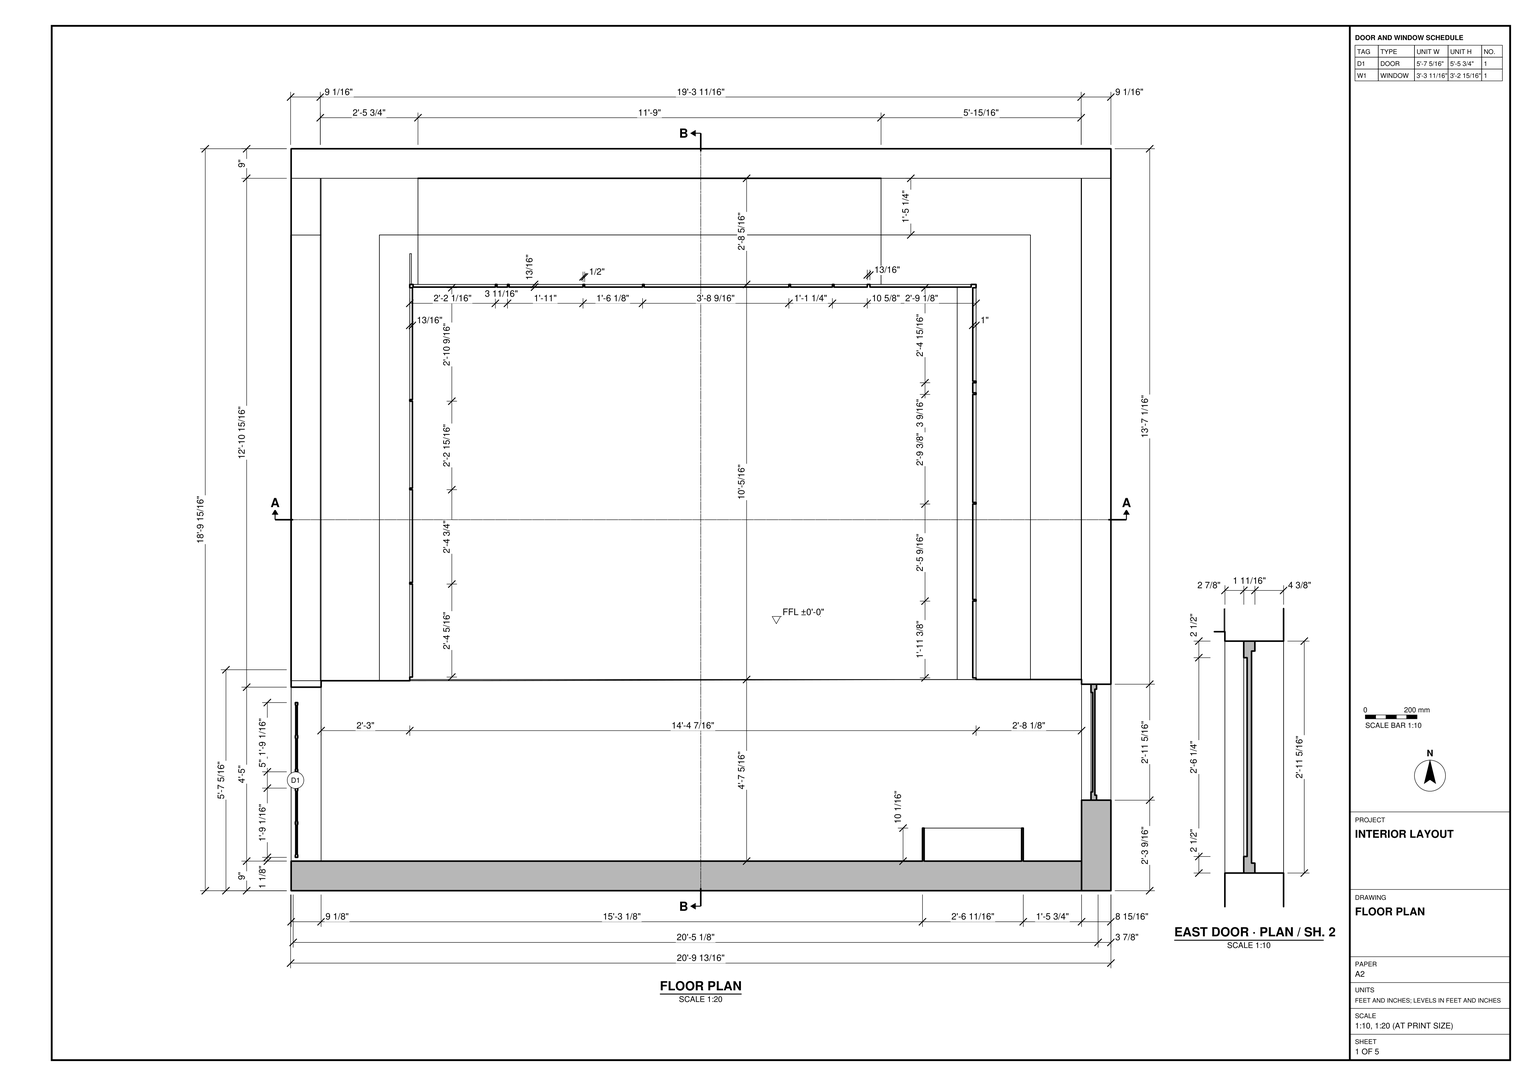
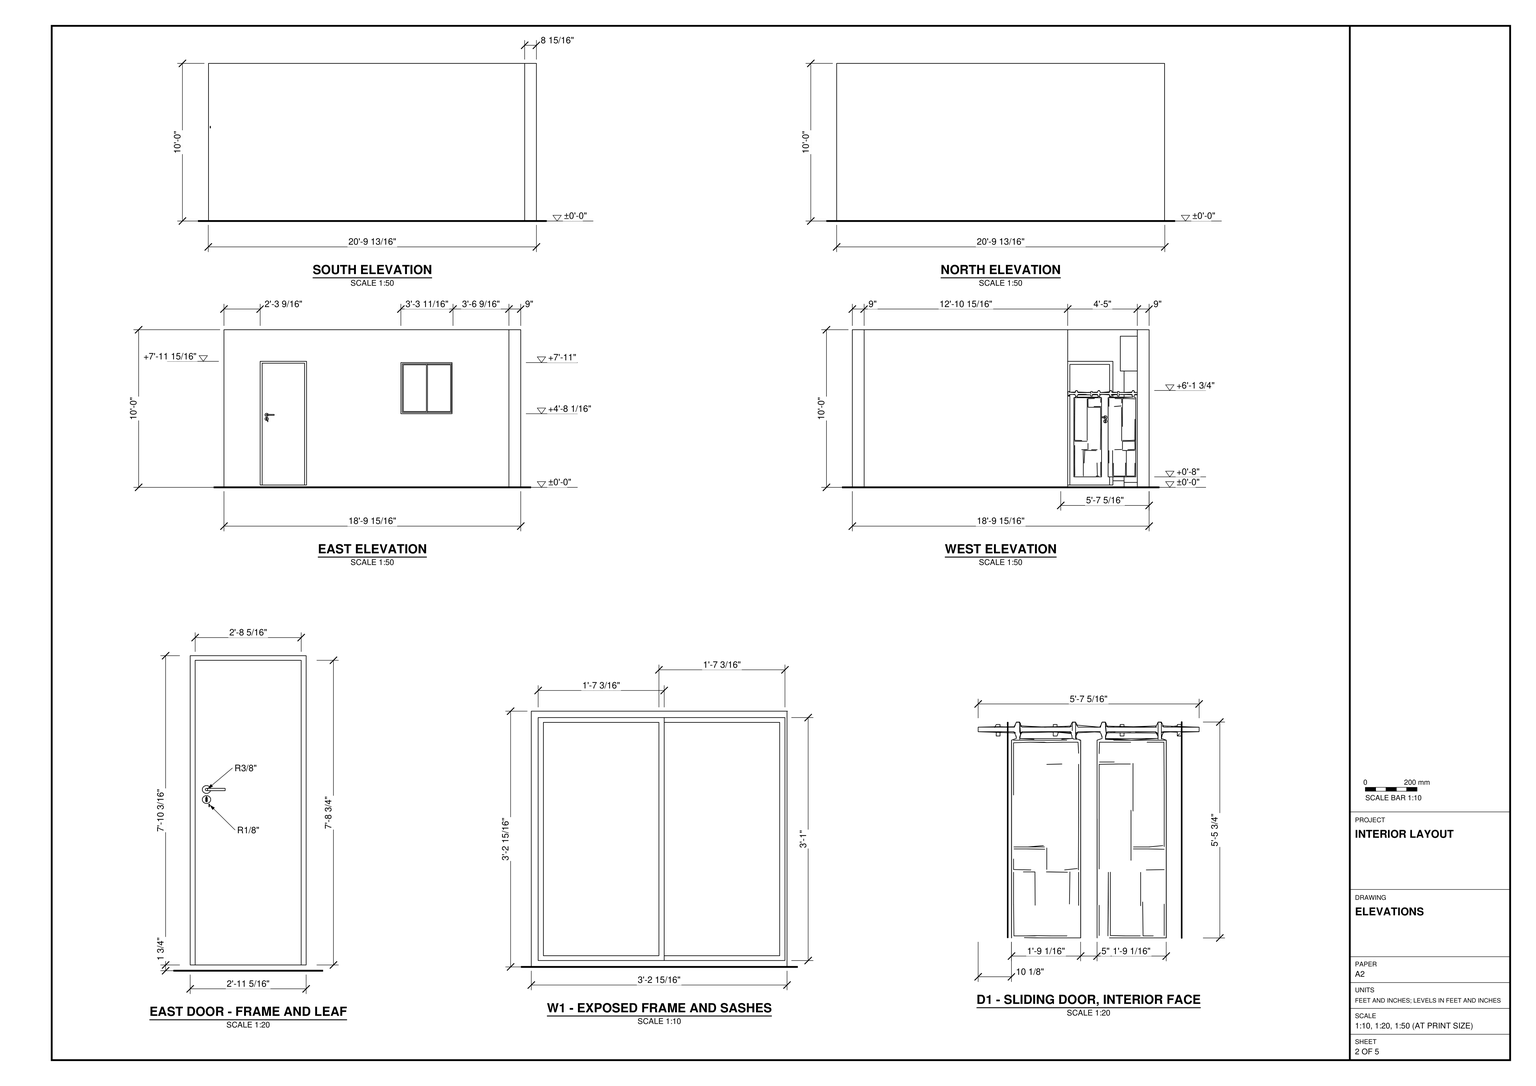
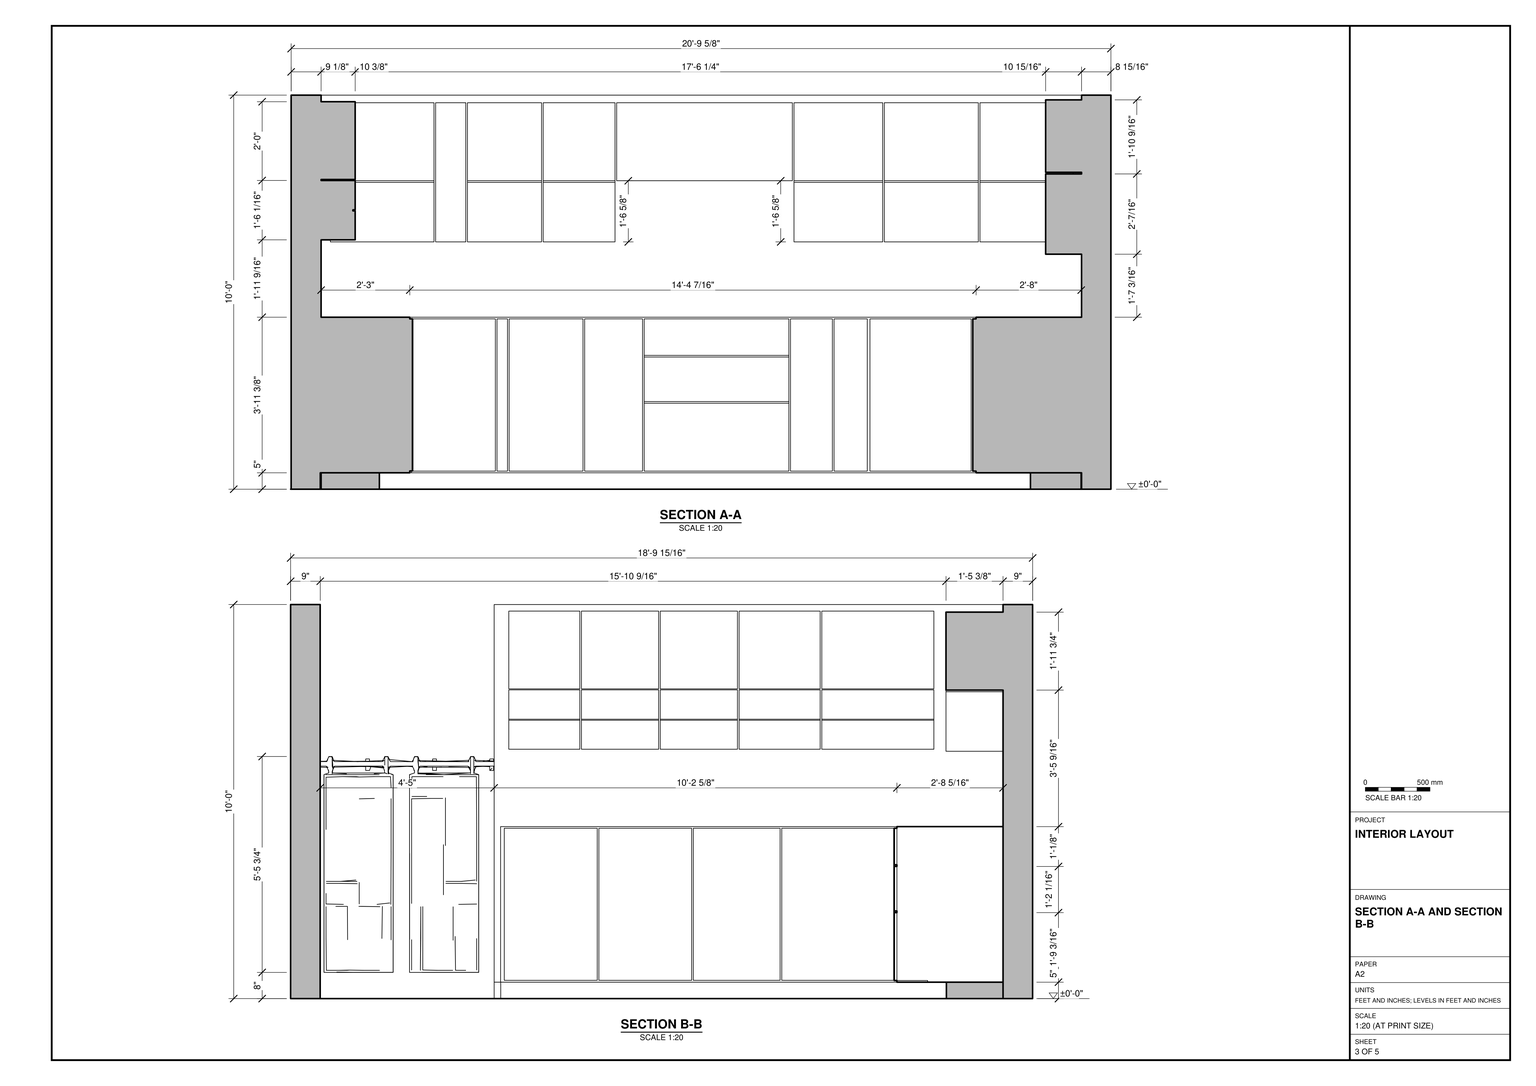
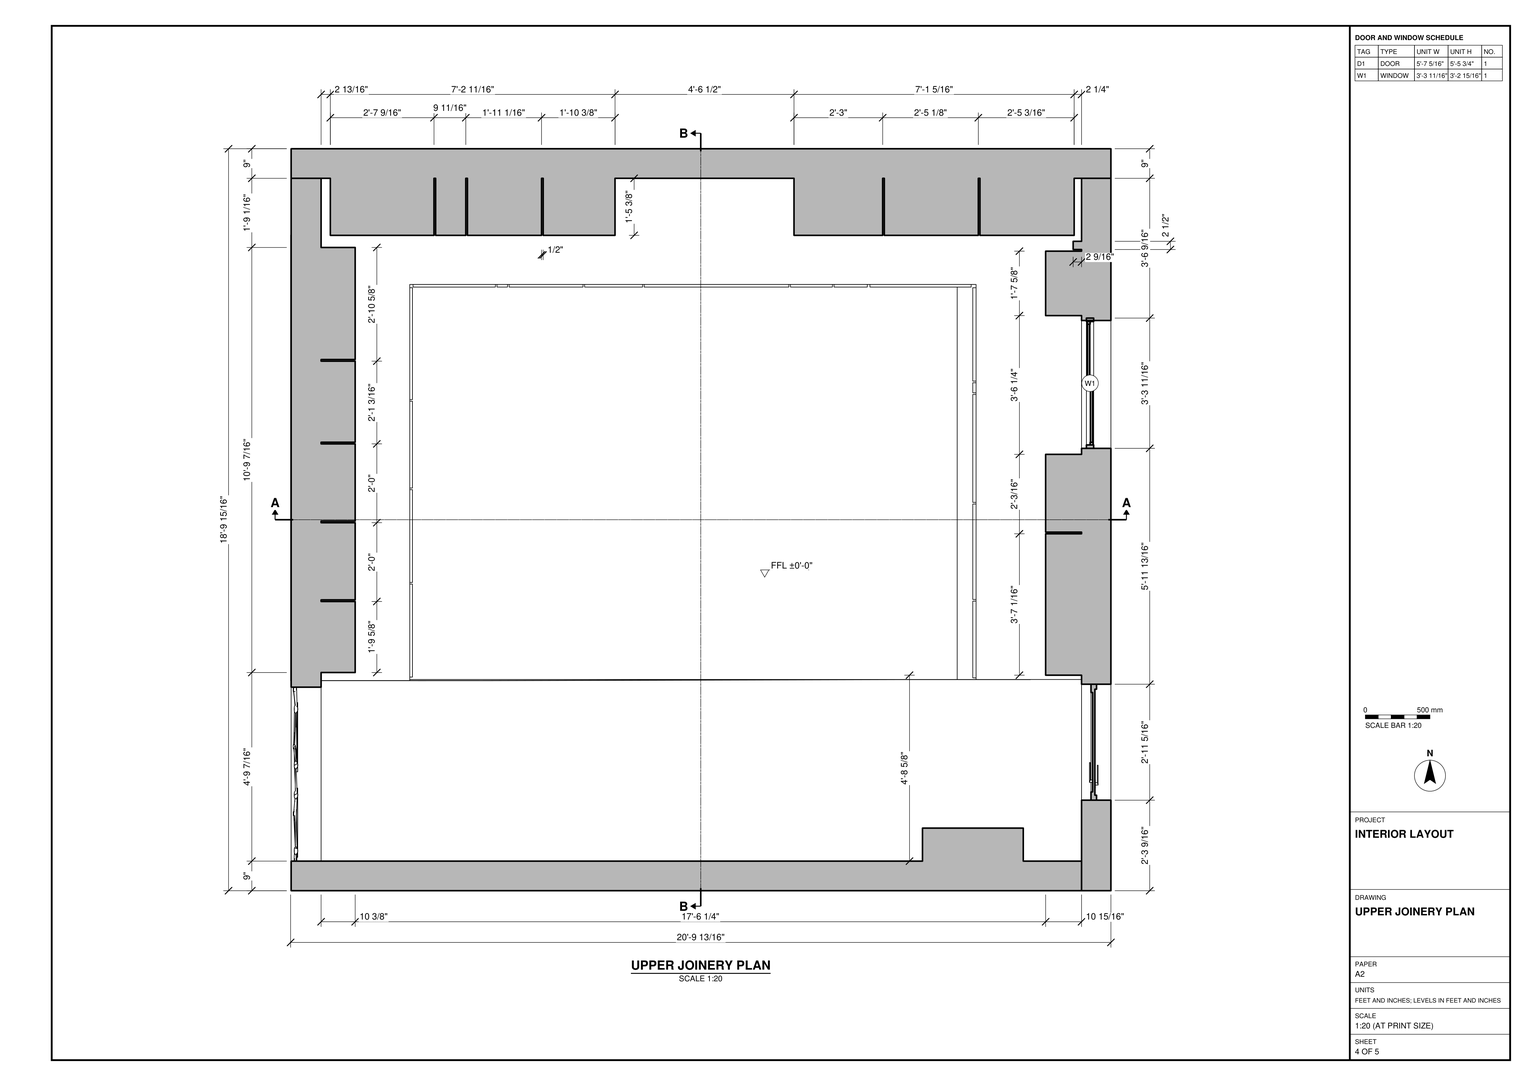
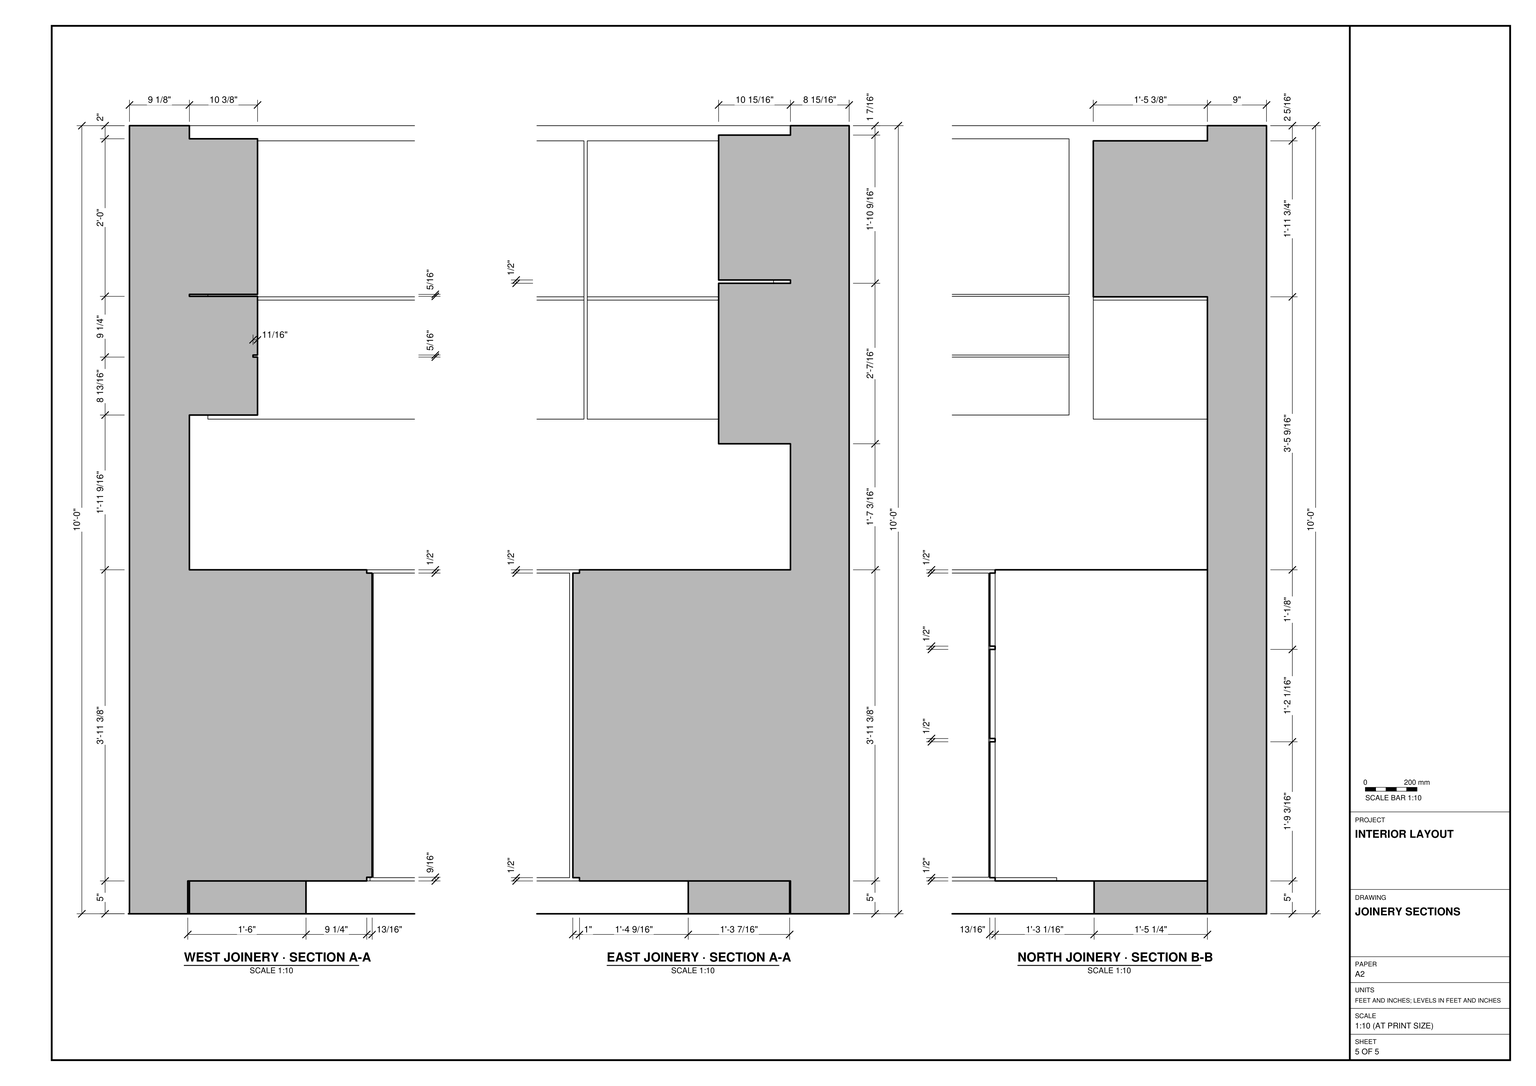
Use task_files/diagram_01.pdf to model the room and its built-in joinery in SketchUp. Work in feet and inches. Set the finished floor at ±0'-0" and make the overall shell 20'-9 13/16" east to west, 18'-9 15/16" north to south and 10'-0" high.

Lay out the perimeter walls at their drawn thicknesses. On the east wall, fit the framed single-leaf door near the south end and the two-sash window farther north. Use the elevation details for the window sill, door frame and hardware. At the south end of the west wall, model the paired sliding panels and their exposed overhead track.

Build the lower cabinetry along the north wall and return it along the west and east walls, leaving the centre open. Use the plan to set out the depths and unequal bay widths. Follow the sections for the raised plinth, lower cabinet fronts, central shelves and wall-mounted storage. Preserve the clear space between the lower and upper units rather than filling it with full-height cabinets.

Keep shell elements and each distinct furniture or joinery piece in separate groups or components. Use components for repeated parts. Any decor or loose items shown may be represented by suitable library components. Save one SketchUp model as output_files/single_room_interior_with_u_shaped_built_in_cabinetry.skp.

# SketchUp Ruby script. Lengths in inches.
U = 1.inch
M = Sketchup.active_model
def pt(a) = Geom::Point3d.new(a.map { |v| v * U })
def face(e, loops, mat)
  f = e.add_face(loops[0].map { |a| pt(a) })
  loops[1..].each { |l| e.add_face(l.map { |a| pt(a) }).erase! }
  f.material = f.back_material = mat if mat
  f
end
# faces: each face lists its corners as indices into pts; further lists are holes
def faces(e, pts, list, mat = nil) = list.each { |f| face(e, (f[0].is_a?(Array) ? f : [f]).map { |l| l.map { |i| pts[i] } }, mat) }
# xy, xz, yz: faces in a plane at the given z, y or x. An outline is a flat list of corners, or four numbers for a rectangle; further outlines are holes
def ring(l) = l.size == 4 ? [[l[0], l[1]], [l[2], l[1]], [l[2], l[3]], [l[0], l[3]]] : l.each_slice(2).to_a
def flat(e, list, mat, &to3) = list.each { |f| face(e, (f[0].is_a?(Array) ? f : [f]).map { |l| ring(l).map { |u, v| to3.(u, v) } }, mat) }
def xy(e, z, list, mat = nil) = flat(e, list, mat) { |x, y| [x, y, z] }
def xz(e, y, list, mat = nil) = flat(e, list, mat) { |x, z| [x, y, z] }
def yz(e, x, list, mat = nil) = flat(e, list, mat) { |y, z| [x, y, z] }
def lines(e, pts, list) = list.each { |a, b| e.add_line(pt(pts[a]), pt(pts[b])) }
# prism: a flat outline (further loops are holes) pulled along v
def prism(e, loops, v, mat = nil)
  f = face(e, loops, mat); d = Geom::Vector3d.new(v.map { |x| x * U })
  f.pushpull(f.normal.samedirection?(d) ? d.length : -d.length)
end
def box(e, o, s, mat = nil) = prism(e, [[o, [o[0] + s[0], o[1], o[2]], [o[0] + s[0], o[1] + s[1], o[2]], [o[0], o[1] + s[1], o[2]]]], [0, 0, s[2]], mat)
def at(x, y, z, deg = 0) = Geom::Transformation.translation(pt([x, y, z])) * Geom::Transformation.rotation(ORIGIN, Z_AXIS, deg.degrees)
def axes(o, x, y, z) = Geom::Transformation.new([*x, 0, *y, 0, *z, 0, *pt(o).to_a, 1])
def part(name) = M.definitions.add(name)
# library, detail: a bought-in or finely detailed component or shape, given as its bounding box
def library(name, o, s) = part(name).tap { |d| box(d.entities, o, s) }
def detail(e, o, s) = box(e.add_group.entities, o, s)
def put(e, d, t, mat = nil) = e.add_instance(d, t).tap { |i| i.material = mat if mat }
def group(e, t, mat = nil) = e.add_group.tap { |g| g.transformation = t; g.material = mat if mat }.entities
root = M.entities
M.materials.add("Wood_Door").color = [227, 177, 138]
M.materials.add("[Color M05]").color = [114, 114, 114]
M.materials.add("[Metal Aluminum Anodized]").color = [202, 209, 219]
M.materials.add("[Metal Corrugated Shiny]").color = [193, 193, 193]
M.materials.add("[Metal Seamed]").color = [118, 119, 115]
M.materials.add("[Translucent Glass Tinted]").color = [1, 25, 30]
M.materials["[Translucent Glass Tinted]"].alpha = 0.31
c1 = part("Group\#98")
g1 = group(c1.entities,at(-0.375,0,0),"[Metal Seamed]")
prism(g1,[[[0.375,0,0],[0.375,0,57],[0.375,26.94,57],[0.375,26.94,0]],[[0.375,25.82,55.875],[0.375,1.125,55.875],[0.375,1.125,1.125],[0.375,25.82,1.125]]],[1.5,0,0])
g2 = group(c1.entities,at(0.18,24.32,1.125),"[Translucent Glass Tinted]")
box(g2,[0,-23.19,0],[1.125,24.69,54.75])
c2 = part("Aluminium+Channel+Glass+Window")
g3 = group(c2.entities,at(-81.68,-4.64,338.57))
g4 = group(g3,at(-22.76,-500.89,-282.52),"[Metal Aluminum Anodized]")
prism(g4,[[[0,0,38.9375],[0,39.67,38.9375],[0,39.67,0],[0,0,0]],[[0,1.05,0.97],[0,38.625,0.97],[0,38.625,37.96],[0,1.05,37.96]]],[2.21,0,0])
put(g3,c1,axes([-22.54,-481.46,-281.55],[0.6,0,0],[0,0.71223,0],[0,0,0.64896]))
put(g3,c1,axes([-21.64,-499.85,-281.55],[0.6,0,0],[0,0.71223,0],[0,0,0.64896]))
c3 = library("Sliding Door 243 092",[-48.06,-2.0625,0.36],[96.12,2.0625,93.93])
c4 = part("Door lever handle")
xz(c4.entities,1.97,[[0.3,0,0.15,0.04,0.04,0.15,0,0.3,0.04,0.44,0.15,0.55,0.3,0.59,0.44,0.55,0.55,0.44,0.59,0.3,0.55,0.15,0.44,0.04]])
yz(c4.entities,4.72,[[0.3,0,0.44,0.04,0.55,0.15,0.59,0.3,0.55,0.44,0.44,0.55,0.3,0.59,0.15,0.55,0.04,0.44,0,0.3,0.04,0.15,0.15,0.04]],"[Metal Corrugated Shiny]")
p = [[0.04,1.97,0.15],[0.15,1.97,0.04],[0.15,0.15,0.04],[0.04,0.04,0.15],[4.72,0.15,0.04],[4.72,0.04,0.15],
  [0.3,1.97,0],[0.3,0.3,0],[4.72,0.3,0],[0.44,1.97,0.04],[0.44,0.44,0.04],[4.72,0.44,0.04],
  [0.55,1.97,0.15],[0.55,0.55,0.15],[4.72,0.55,0.15],[0,1.97,0.3],[0,0,0.3],[4.72,0,0.3],
  [0.59,1.97,0.3],[0.59,0.59,0.3],[4.72,0.59,0.3],[0.04,1.97,0.44],[0.04,0.04,0.44],[4.72,0.04,0.44],
  [0.55,1.97,0.44],[0.55,0.55,0.44],[4.72,0.55,0.44],[0.15,1.97,0.55],[0.15,0.15,0.55],[4.72,0.15,0.55],
  [0.44,1.97,0.55],[0.44,0.44,0.55],[4.72,0.44,0.55],[0.3,1.97,0.59],[0.3,0.3,0.59],[4.72,0.3,0.59]]
faces(c4.entities,p,[[0,1,2,3],[3,2,4,5],[1,6,7,2],[2,7,8,4],[6,9,10,7],[7,10,11,8],[9,12,13,10],[10,13,14,11],
  [15,0,3,16],[16,3,5,17],[12,18,19,13],[13,19,20,14],[21,15,16,22],[22,16,17,23],[18,24,25,19],[19,25,26,20],
  [27,21,22,28],[28,22,23,29],[24,30,31,25],[25,31,32,26],[33,27,28,34],[34,28,29,35],[30,33,34,31],[31,34,35,32]],"[Metal Corrugated Shiny]")
c5 = part("Door handle rose")
xy(c5.entities,0,[[0.72,0,1.25,0.31]],"[Metal Corrugated Shiny]")
xy(c5.entities,1.97,[[0.72,0,1.25,0.31]],"[Metal Corrugated Shiny]")
xz(c5.entities,0,[[0.72,0,1.25,0,1.71,0.26,1.97,0.72,1.97,1.25,1.71,1.71,1.25,1.97,0.72,1.97,0.26,1.71,0,1.25,0,0.72,0.26,0.26]],"[Metal Corrugated Shiny]")
yz(c5.entities,0,[[0,0.72,0.31,1.25]],"[Metal Corrugated Shiny]")
yz(c5.entities,1.97,[[0,0.72,0.31,1.25]],"[Metal Corrugated Shiny]")
p = [[0.26,0.31,0.26],[0.72,0.31,0],[0.72,0,0],[0.26,0,0.26],[1.25,0.31,0],[1.71,0.31,0.26],
  [1.71,0,0.26],[1.25,0,0],[0,0.31,0.72],[0,0,0.72],[1.97,0.31,0.72],[1.97,0,0.72],
  [0.26,0.31,1.71],[0,0.31,1.25],[0,0,1.25],[0.26,0,1.71],[1.97,0.31,1.25],[1.71,0.31,1.71],
  [1.71,0,1.71],[1.97,0,1.25],[0.72,0.31,1.97],[0.72,0,1.97],[1.25,0.31,1.97],[1.25,0,1.97]]
faces(c5.entities,p,[[0,1,2,3],[4,5,6,7],[8,0,3,9],[5,10,11,6],[12,13,14,15],[16,17,18,19],[20,12,15,21],[17,22,23,18]],"[Metal Corrugated Shiny]")
c6 = part("Small_Key")
xy(c6.entities,0,[[0.06,2.125,0.18,2.52]],"[Metal Corrugated Shiny]")
xy(c6.entities,0.1,[[0.06,0,0.18,0.63]],"[Metal Corrugated Shiny]")
xy(c6.entities,0.26,[[0.06,0.16,0.18,0.47]],"[Metal Corrugated Shiny]")
xy(c6.entities,0.89,[[0.06,0.16,0.18,0.47]],"[Metal Corrugated Shiny]")
xy(c6.entities,1.05,[[0.06,0,0.18,0.63]],"[Metal Corrugated Shiny]")
xz(c6.entities,0,[[0.06,0.1,0.18,1.05]],"[Metal Corrugated Shiny]")
xz(c6.entities,0.16,[[0.06,0.26,0.18,0.89]],"[Metal Corrugated Shiny]")
xz(c6.entities,0.47,[[0.06,0.26,0.18,0.89]],"[Metal Corrugated Shiny]")
xz(c6.entities,0.63,[[0.06,0.1,0.06,0.47,0.12,0.46,0.18,0.47,0.18,0.1],[0.06,0.68,0.06,1.05,0.18,1.05,0.18,0.68,0.12,0.69]],"[Metal Corrugated Shiny]")
xz(c6.entities,2.125,[[0.06,0,0.18,0,0.18,0.47,0.12,0.46,0.06,0.47]],"[Metal Corrugated Shiny]")
xz(c6.entities,2.52,[[0.06,0,0.06,0.47,0.12,0.46,0.18,0.47,0.18,0]],"[Metal Corrugated Shiny]")
xz(c6.entities,2.6,[[0.12,0.46,0.06,0.47,0.02,0.52,0,0.57,0.02,0.63,0.06,0.68,0.12,0.69,0.18,0.68,0.22,0.63,0.24,0.57,0.22,0.52,0.18,0.47]],"[Metal Corrugated Shiny]")
yz(c6.entities,0.06,[[2.125,0,2.52,0.47],[[0,0.1,0.63,1.05],[0.16,0.26,0.47,0.89]]],"[Metal Corrugated Shiny]")
yz(c6.entities,0.18,[[2.125,0,2.52,0.47],[[0,0.1,0.63,1.05],[0.16,0.26,0.47,0.89]]],"[Metal Corrugated Shiny]")
p = [[0.06,2.6,0.47],[0.06,2.52,0.47],[0.06,2.125,0.47],[0.06,0.63,0.47],[0.04,0.6875,0.49],[0.02,0.72,0.52],
  [0.02,2.6,0.52],[0.04,0.6875,0.66],[0.06,0.63,0.68],[0.12,0.63,0.46],[0.12,2.125,0.46],[0.18,2.125,0.47],
  [0.18,0.63,0.47],[0.22,2.6,0.52],[0.22,0.72,0.52],[0.19,0.6875,0.49],[0.18,2.52,0.47],[0.18,2.6,0.47],
  [0.19,0.6875,0.66],[0.18,0.63,0.68],[0.02,0.72,0.63],[0,0.73,0.57],[0,2.6,0.57],[0.24,0.73,0.57],
  [0.22,0.72,0.63],[0.24,2.6,0.57],[0.12,2.52,0.46],[0.12,2.6,0.46],[0.02,2.6,0.63],[0.06,2.6,0.68],
  [0.18,2.6,0.68],[0.22,2.6,0.63],[0.12,2.6,0.69],[0.12,0.63,0.69]]
faces(c6.entities,p,[[0,1,2,3,4,5,6],[7,4,3,8],[9,10,11,12],[3,2,10,9],[13,14,15,12,11,16,17],[15,18,19,12],[20,21,5,4,7],[6,5,21,22],
  [14,23,24,18,15],[25,23,14,13],[10,26,16,11],[2,1,26,10],[27,17,16,26],[0,27,26,1],[28,20,7,8,29],[30,19,18,24,31],
  [22,21,20,28],[31,24,23,25],[30,32,33,19],[32,29,8,33]],"[Metal Corrugated Shiny]")
c7 = part("Lock key")
put(c7.entities,c6,at(0.08,-1.14,0.29))
c8 = part("lock")
xy(c8.entities,0.12,[[0.1,0.24,0.3,0.28]],"[Color M05]")
xz(c8.entities,0.28,[[0.1,0.12,0.3,0.12,0.3,0.7,0.37,0.77,0.39,0.87,0.37,0.96,0.3,1.04,0.2,1.0625,0.1,1.04,0.03,0.96,0,0.87,0.03,0.77,0.1,0.7]],"[Color M05]")
yz(c8.entities,0,[[0,0.2,0.24,0.98]],"[Color M05]")
yz(c8.entities,0.1,[[0.24,0.12,0.28,0.7]],"[Color M05]")
yz(c8.entities,0.3,[[0.24,0.12,0.28,0.7]],"[Color M05]")
yz(c8.entities,0.39,[[0,0.2,0.24,0.98]],"[Color M05]")
p = [[0.03,0,0.1],[0.1,0,0.03],[0.1,0.24,0.03],[0.03,0.24,0.1],[0.2,0,0],[0.2,0.24,0],
  [0.3,0,0.03],[0.3,0.24,0.03],[0.37,0,0.1],[0.37,0.24,0.1],[0,0,0.2],[0,0.24,0.2],
  [0.39,0,0.2],[0.39,0.24,0.2],[0.03,0.24,0.77],[0.1,0.24,0.7],[0.1,0.28,0.7],[0.03,0.28,0.77],
  [0.3,0.24,0.7],[0.37,0.24,0.77],[0.37,0.28,0.77],[0.3,0.28,0.7],[0,0.24,0.87],[0,0.28,0.87],
  [0.39,0.24,0.87],[0.39,0.28,0.87],[0.03,0.24,0.96],[0.03,0.28,0.96],[0.37,0.24,0.96],[0.37,0.28,0.96],
  [0.03,0,1.08],[0,0,0.98],[0,0.24,0.98],[0.03,0.24,1.08],[0.39,0,0.98],[0.37,0,1.08],
  [0.37,0.24,1.08],[0.39,0.24,0.98],[0.1,0.24,1.04],[0.1,0.28,1.04],[0.2,0.24,1.0625],[0.2,0.28,1.0625],
  [0.3,0.24,1.04],[0.3,0.28,1.04],[0.1,0,1.15],[0.1,0.24,1.15],[0.3,0,1.15],[0.3,0.24,1.15],
  [0.2,0,1.18],[0.2,0.24,1.18]]
faces(c8.entities,p,[[0,1,2,3],[1,4,5,2],[4,6,7,5],[6,8,9,7],[10,0,3,11],[8,12,13,9],[14,15,16,17],[18,19,20,21],
  [22,14,17,23],[19,24,25,20],[26,22,23,27],[24,28,29,25],[30,31,32,33],[34,35,36,37],[38,26,27,39],[40,38,39,41],
  [42,40,41,43],[28,42,43,29],[44,30,33,45],[35,46,47,36],[48,44,45,49],[46,48,49,47]],"[Color M05]")
put(c8.entities,c7,at(0,0,0))
c9 = part("Group\#78")
put(c9.entities,c4,at(0.6875,0.39,3.25))
put(c9.entities,c5,axes([0,2.36,2.56],[0.99853,0,0],[0,1,0],[0,0,0.99853]),"[Metal Corrugated Shiny]")
g5 = group(c9.entities,at(0,2.36,-0.39))
xy(g5,0.39,[[0.72,0,1.25,0.31]],"[Metal Corrugated Shiny]")
xy(g5,2.36,[[0.72,0,1.25,0.31]],"[Metal Corrugated Shiny]")
xz(g5,0,[[[0.72,0.39,1.25,0.39,1.7,0.66,1.97,1.11,1.97,1.64,1.7,2.1,1.25,2.36,0.72,2.36,0.26,2.1,0,1.64,0,1.11,0.26,0.66],[0.98,0.79,0.89,0.8125,0.8125,0.89,0.79,0.98,0.79,1.77,0.8125,1.87,0.89,1.94,0.98,1.97,1.08,1.94,1.15,1.87,1.18,1.77,1.18,0.98,1.15,0.89,1.08,0.8125]]],"[Metal Corrugated Shiny]")
yz(g5,0,[[0,1.11,0.31,1.64]],"[Metal Corrugated Shiny]")
yz(g5,1.97,[[0,1.11,0.31,1.64]],"[Metal Corrugated Shiny]")
p = [[0.26,0.31,0.66],[0.72,0.31,0.39],[0.72,0,0.39],[0.26,0,0.66],[1.25,0.31,0.39],[1.7,0.31,0.66],
  [1.7,0,0.66],[1.25,0,0.39],[0,0.31,1.11],[0,0,1.11],[1.97,0.31,1.11],[1.97,0,1.11],
  [0.26,0.31,2.1],[0,0.31,1.64],[0,0,1.64],[0.26,0,2.1],[1.97,0.31,1.64],[1.7,0.31,2.1],
  [1.7,0,2.1],[1.97,0,1.64],[0.72,0.31,2.36],[0.72,0,2.36],[1.25,0.31,2.36],[1.25,0,2.36]]
faces(g5,p,[[0,1,2,3],[4,5,6,7],[8,0,3,9],[5,10,11,6],[12,13,14,15],[16,17,18,19],[20,12,15,21],[17,22,23,18]],"[Metal Corrugated Shiny]")
g6 = group(c9.entities,at(0.79,2.36,0.39))
put(g6,c8,at(0,0,0))
c10 = part("door+(2)")
put(c10.entities,c3,axes([124.66,468.18,7.72],[0.7,0,0],[0,0.7,0],[0,0,0.7]))
g7 = group(c10.entities,at(118.58,223.07,1.75))
xy(g7,0,[[0,0.47,0,2.17,2.52,2.17,2.52,1.66,32.79,1.66,32.79,2.17,35.3125,2.17,35.3125,0.47,33.8,0.47,33.8,0.98,1.51,0.98,1.51,0.47]])
xy(g7,91.83,[[2.52,1.66,32.79,2.17]],"Wood_Door")
xy(g7,92.77,[[1.51,0.47,33.8,0.98]],"Wood_Door")
xy(g7,94.1875,[[0,0.47,35.3125,2.17]],"Wood_Door")
xz(g7,0.47,[[0,0,1.51,0,1.51,92.77,33.8,92.77,33.8,0,35.3125,0,35.3125,94.1875,0,94.1875]],"Wood_Door")
xz(g7,0.98,[[1.51,0,33.8,92.77]],"Wood_Door")
xz(g7,1.66,[[2.52,0,32.79,91.83]])
xz(g7,2.17,[[0,0,0,94.1875,35.3125,94.1875,35.3125,0,32.79,0,32.79,91.83,2.52,91.83,2.52,0]])
yz(g7,0,[[0.47,0,2.17,94.1875]],"Wood_Door")
yz(g7,1.51,[[0.47,0,0.98,92.77]],"Wood_Door")
yz(g7,2.52,[[1.66,0,2.17,91.83]],"Wood_Door")
yz(g7,32.79,[[1.66,0,2.17,91.83]],"Wood_Door")
yz(g7,33.8,[[0.47,0,0.98,92.77]],"Wood_Door")
yz(g7,35.3125,[[0.47,0,2.17,94.1875]],"Wood_Door")
p = [[32.79,2.17,0],[2.52,2.17,0]]
lines(g7,p,[[0,1]])
put(g7,c9,axes([3.71,-0.17,49.2],[1.28134,0,0],[0,0.43,0],[0,0,1.19618]))
put(g7,c9,axes([4.52,2.81,47.34],[1.28134,0,0],[0,-0.43,0],[0,0,1.19618]))
xy(root,0,[[0.16,0,9.29,9],[9.29,0,9.29,9,192.41,9,192.41,19.0625,223.1,19.0625,223.1,9,240.85,9,240.85,0],[240.85,0,249.79,216.9375],[0.16,9,9.29,61.97],[9.29,9,192.41,9,192.41,19.0625,223.1,19.0625,223.1,9,240.85,9,240.85,64.3125,225.29,64.3125,225.29,64.27,202.98,64.27,202.98,64.3125,179.79,64.3125,38.79,63.9375,9.29,63.9375],
  [0.16,61.97,9.29,216.9375],[9.29,63.9375,38.79,63.9375,179.79,64.3125,9.29,64.3125],[202.98,64.27,225.29,64.3125],[9.29,64.3125,202.98,64.3125,202.98,199.6875,225.29,199.6875,225.29,64.3125,240.85,64.3125,240.85,216.9375,9.29,216.9375],[202.98,64.3125,225.29,199.6875],
  [0.16,216.9375,249.79,225.9375]])
xy(root,1.75,[[240.85,27.5625,249.79,62.875]])
xy(root,5,[[9.29,63.9375,9.29,216.9375,38.79,216.9375,38.79,184.62,36.79,184.62,36.79,193.99,36.29,193.99,36.29,63.9375],[208.72,64.3125,208.72,184.62,179.79,184.62,179.79,216.9375,240.85,216.9375,240.85,64.3125],[38.79,184.62,179.79,216.9375]])
xy(root,5.5,[[207.72,64.8125,208.72,88.18],[207.72,88.68,208.72,117.74],[207.72,118.24,208.72,151.12],[207.72,151.62,208.72,154.68],[207.72,155.18,208.72,183.62],
  [37.29,183.8,62.35,184.62],[62.85,183.8,66.04,184.62],[66.54,183.8,89.04,184.62],[89.54,183.8,107.16,184.62],[107.66,183.8,151.72,184.62],
  [152.22,183.8,164.97,184.62],[165.47,183.8,175.6,184.62],[176.41,183.8,207.22,184.62],[36.29,184.62,36.79,193.99]])
xy(root,5.5625,[[36.29,65.05,37.1,93.37],[36.29,93.87,37.1,122.12],[36.29,122.62,37.1,149.05],[36.29,149.55,37.1,183.62]])
xy(root,26.1875,[[107.66,183.8,151.72,184.62]])
xy(root,26.6875,[[107.66,183.8,151.72,184.62]])
xy(root,35.5625,[[192.91,9,222.6,19.0625]])
xy(root,40.25,[[107.66,183.8,151.72,184.62]])
xy(root,40.75,[[107.66,183.8,151.72,184.62]])
xy(root,51.875,[[207.72,64.8125,208.72,88.18],[36.29,65.05,37.1,93.37],[207.72,88.68,208.72,117.74],[36.29,93.87,37.1,122.12],[207.72,118.24,208.72,151.12],
  [36.29,122.62,37.1,149.05],[36.29,149.55,37.1,183.62],[207.72,151.62,208.72,154.68],[207.72,155.18,208.72,183.62],[37.29,183.8,62.35,184.62],
  [62.85,183.8,66.04,184.62],[66.54,183.8,89.04,184.62],[89.54,183.8,107.16,184.62],[107.66,183.8,151.72,184.62],[152.22,183.8,164.97,184.62],
  [165.47,183.8,175.6,184.62],[176.41,183.8,207.22,184.62]])
xy(root,52.375,[[9.29,63.9375,36.29,63.9375,36.29,184.62,208.72,184.62,208.72,64.3125,240.85,64.3125,240.85,216.9375,9.29,216.9375]])
xy(root,56.05,[[240.85,134.7,249.79,173.63]])
xy(root,62.0625,[[192.91,9,222.6,19.0625]])
xy(root,71.5625,[[229.91,65.625,240.85,108.6875],[229.91,109.1875,240.85,132.875],[229.91,175.125,240.85,194.75],[238.29,195.25,240.85,197.75]])
xy(root,75.3125,[[12.1,199.5625,43.66,216.9375],[44.16,199.5625,53.35,216.9375],[53.85,199.5625,76.41,216.9375],[76.91,199.5625,98.79,216.9375],[153.29,199.5625,180.29,216.9375],
  [180.79,199.5625,209.41,216.9375],[209.91,199.5625,238.6,216.9375]])
xy(root,75.9375,[[9.29,66.4375,19.66,88.0625],[9.29,88.5625,19.66,112.0625],[9.29,112.5625,19.66,136.0625],[9.29,136.5625,19.66,161.25],[9.29,161.75,19.66,195.875]])
xy(root,84.76,[[18.97,66.4375,19.66,88.0625],[18.97,88.5625,19.66,112.0625],[18.97,112.5625,19.66,136.0625],[18.97,136.5625,19.66,161.25],[18.6,161.75,19.66,195.875]])
xy(root,85.08,[[18.97,66.4375,19.66,88.0625],[18.97,88.5625,19.66,112.0625],[18.97,112.5625,19.66,136.0625],[18.97,136.5625,19.66,161.25],[18.6,161.75,19.66,195.875]])
xy(root,88.5625,[[192.91,8.4375,222.6,19.0625],[132.91,9,161.91,21.9375],[162.41,9,191.91,21.9375]])
xy(root,93.4375,[[12.1,199.5625,43.66,216.9375],[53.85,199.5625,76.41,216.9375],[76.91,199.5625,98.79,216.9375],[153.29,199.5625,180.29,216.9375],[180.79,199.5625,209.41,216.9375],
  [209.91,199.5625,238.6,216.9375]])
xy(root,93.9375,[[12.1,199.5625,43.66,216.9375],[53.85,199.5625,76.41,216.9375],[76.91,199.5625,98.79,216.9375],[99.29,199.5625,152.79,216.9375],[153.29,199.5625,180.29,216.9375],
  [180.79,199.5625,209.41,216.9375],[209.91,199.5625,238.6,216.9375]])
xy(root,94.01,[[9.29,66.4375,19.66,88.0625],[9.29,88.5625,19.66,112.0625],[9.29,112.5625,19.66,136.0625],[9.29,136.5625,19.66,161.25],[9.29,161.75,19.66,195.875]])
xy(root,94.3125,[[9.29,66.4375,19.66,88.0625],[9.29,88.5625,19.66,112.0625],[9.29,112.5625,19.66,136.0625],[9.29,136.5625,19.66,161.25],[9.29,161.75,19.66,195.875]])
xy(root,94.98,[[240.85,134.7,249.79,173.63]])
xy(root,95.9375,[[240.85,27.5625,249.79,62.875]])
xy(root,96,[[229.91,65.625,240.85,108.6875],[229.91,109.1875,240.85,132.875],[229.91,175.125,240.85,194.75]])
xy(root,96.5,[[229.91,65.625,240.85,108.6875],[229.91,109.1875,240.85,126.5],[229.91,127,240.85,153.3125],[229.91,153.8125,240.85,178.875],[229.91,179.375,240.85,194.75]])
xy(root,114.5625,[[192.91,8.4375,222.6,19.0625]])
xy(root,115.0625,[[132.91,9,161.91,21.9375],[162.41,9,191.91,21.9375],[192.41,9,222.6,19.0625],[222.6,9,223.1,19.0625]])
xy(root,117.6875,[[12.1,199.5625,43.66,216.9375],[44.16,199.5625,53.35,216.9375],[53.85,199.5625,76.41,216.9375],[76.91,199.5625,98.79,216.9375],[99.29,199.5625,152.79,216.9375],
  [153.29,199.5625,180.29,216.9375],[180.79,199.5625,209.41,216.9375],[209.91,199.5625,238.6,216.9375]])
xy(root,118,[[9.29,66.4375,19.66,88.0625],[9.29,88.5625,19.66,112.0625],[9.29,112.5625,19.66,136.0625],[9.29,136.5625,19.66,161.25],[9.29,161.75,19.66,195.875]])
xy(root,118.5625,[[229.91,65.625,240.85,108.6875],[229.91,109.1875,240.85,126.5],[229.91,127,240.85,153.3125],[229.91,153.8125,240.85,178.875],[229.91,179.375,240.85,194.75],
  [238.29,195.25,240.85,197.75]])
xy(root,120,[[0.16,0,240.85,9],[240.85,0,249.79,216.9375],[0.16,61.97,9.29,66.47],[0.16,66.47,9.29,216.9375],[0.16,216.9375,249.79,225.9375]])
xz(root,0,[[0.16,0,240.85,120],[240.85,0,249.79,120]])
xz(root,8.4375,[[192.91,88.5625,222.6,114.5625]])
xz(root,9,[[0.16,0,9.29,120],[[9.29,0,9.29,120,240.85,120,240.85,0,223.1,0,223.1,115.0625,192.41,115.0625,192.41,0],[162.41,88.5625,191.91,115.0625],[132.91,88.5625,161.91,115.0625]],[192.91,35.5625,222.6,62.0625]])
xz(root,19.0625,[[[192.41,0,192.41,115.0625,223.1,115.0625,223.1,0,222.6,0,222.6,35.0625,192.91,35.0625,192.91,0],[192.91,35.5625,222.6,88.0625],[192.91,88.5625,222.6,114.5625]],[192.91,0,222.6,35.0625],[192.91,62.0625,222.6,88.0625]])
xz(root,21.9375,[[132.91,88.5625,161.91,115.0625],[162.41,88.5625,191.91,115.0625]])
xz(root,27.5625,[[240.85,1.75,249.79,5],[240.85,5,249.79,95.9375]])
xz(root,61.97,[[0.16,0,9.29,120]])
xz(root,62.875,[[240.85,1.75,249.79,5],[240.85,5,249.79,95.9375]])
xz(root,63.9375,[[9.29,5,36.29,52.375]])
xz(root,64.3125,[[208.72,5,240.85,52.375]])
xz(root,64.8125,[[207.72,5.5,208.72,51.875]])
xz(root,65.05,[[36.29,5.5625,37.1,51.875]])
xz(root,65.625,[[229.91,71.5625,240.85,96],[229.91,96.5,240.85,118.5625]])
xz(root,66.4375,[[9.29,75.9375,19.66,75.9375,19.66,84.76,18.97,84.76,18.97,85.08,19.66,85.08,19.66,94.01,9.29,94.01],[9.29,94.3125,19.66,118]])
xz(root,88.0625,[[9.29,75.9375,9.29,94.01,19.66,94.01,19.66,85.08,18.97,85.08,18.97,84.76,19.66,84.76,19.66,75.9375],[9.29,94.3125,19.66,118]])
xz(root,88.18,[[207.72,5.5,208.72,51.875]])
xz(root,88.5625,[[9.29,75.9375,19.66,75.9375,19.66,84.76,18.97,84.76,18.97,85.08,19.66,85.08,19.66,94.01,9.29,94.01],[9.29,94.3125,19.66,118]])
xz(root,88.68,[[207.72,5.5,208.72,51.875]])
xz(root,93.37,[[36.29,5.5625,37.1,51.875]])
xz(root,93.87,[[36.29,5.5625,37.1,51.875]])
xz(root,108.6875,[[229.91,71.5625,240.85,96],[229.91,96.5,240.85,118.5625]])
xz(root,109.1875,[[229.91,71.5625,240.85,96],[229.91,96.5,240.85,118.5625]])
xz(root,112.0625,[[9.29,75.9375,9.29,94.01,19.66,94.01,19.66,85.08,18.97,85.08,18.97,84.76,19.66,84.76,19.66,75.9375],[9.29,94.3125,19.66,118]])
xz(root,112.5625,[[9.29,75.9375,19.66,75.9375,19.66,84.76,18.97,84.76,18.97,85.08,19.66,85.08,19.66,94.01,9.29,94.01],[9.29,94.3125,19.66,118]])
xz(root,117.74,[[207.72,5.5,208.72,51.875]])
xz(root,118.24,[[207.72,5.5,208.72,51.875]])
xz(root,122.12,[[36.29,5.5625,37.1,51.875]])
xz(root,122.62,[[36.29,5.5625,37.1,51.875]])
xz(root,126.5,[[229.91,96.5,240.85,118.5625]])
xz(root,127,[[229.91,96.5,240.85,118.5625]])
xz(root,132.875,[[229.91,71.5625,240.85,96]])
xz(root,134.7,[[240.85,56.05,249.79,94.98]])
xz(root,136.0625,[[9.29,75.9375,9.29,94.01,19.66,94.01,19.66,85.08,18.97,85.08,18.97,84.76,19.66,84.76,19.66,75.9375],[9.29,94.3125,19.66,118]])
xz(root,136.5625,[[9.29,75.9375,19.66,75.9375,19.66,84.76,18.97,84.76,18.97,85.08,19.66,85.08,19.66,94.01,9.29,94.01],[9.29,94.3125,19.66,118]])
xz(root,149.05,[[36.29,5.5625,37.1,51.875]])
xz(root,149.55,[[36.29,5.5625,37.1,51.875]])
xz(root,151.12,[[207.72,5.5,208.72,51.875]])
xz(root,151.62,[[207.72,5.5,208.72,51.875]])
xz(root,153.3125,[[229.91,96.5,240.85,118.5625]])
xz(root,153.8125,[[229.91,96.5,240.85,118.5625]])
xz(root,154.68,[[207.72,5.5,208.72,51.875]])
xz(root,155.18,[[207.72,5.5,208.72,51.875]])
xz(root,161.25,[[9.29,75.9375,9.29,94.01,19.66,94.01,19.66,85.08,18.97,85.08,18.97,84.76,19.66,84.76,19.66,75.9375],[9.29,94.3125,19.66,118]])
xz(root,161.75,[[9.29,75.9375,19.66,75.9375,19.66,84.76,18.6,84.76,18.6,85.08,19.66,85.08,19.66,94.01,9.29,94.01],[9.29,94.3125,19.66,118]])
xz(root,173.63,[[240.85,56.05,249.79,94.98]])
xz(root,175.125,[[229.91,71.5625,240.85,96]])
xz(root,178.875,[[229.91,96.5,240.85,118.5625]])
xz(root,179.375,[[229.91,96.5,240.85,118.5625]])
xz(root,183.62,[[207.72,5.5,208.72,51.875],[36.29,5.5625,37.1,51.875]])
xz(root,183.8,[[37.29,5.5,62.35,51.875],[62.85,5.5,66.04,51.875],[66.54,5.5,89.04,51.875],[89.54,5.5,107.16,51.875],[107.66,5.5,151.72,26.1875],
  [152.22,5.5,164.97,51.875],[165.47,5.5,175.6,51.875],[176.41,5.5,207.22,51.875],[107.66,26.6875,151.72,40.25],[107.66,40.75,151.72,51.875]])
xz(root,184.62,[[[36.79,5,208.72,5,208.72,52.375,36.29,52.375,36.29,5.5,36.79,5.5],[107.66,5.5,151.72,51.875],[176.41,5.5,207.22,51.875],[37.29,5.5,62.35,51.875],[66.54,5.5,89.04,51.875],[89.54,5.5,107.16,51.875],[152.22,5.5,164.97,51.875],[165.47,5.5,175.6,51.875],[62.85,5.5,66.04,51.875]],[107.66,26.1875,151.72,26.6875],[107.66,40.25,151.72,40.75]])
xz(root,193.99,[[36.29,5,36.79,5.5]])
xz(root,194.75,[[229.91,71.5625,240.85,96],[229.91,96.5,240.85,118.5625]])
xz(root,195.25,[[238.29,71.5625,240.85,118.5625]])
xz(root,195.875,[[9.29,75.9375,9.29,94.01,19.66,94.01,19.66,85.08,18.6,85.08,18.6,84.76,19.66,84.76,19.66,75.9375],[9.29,94.3125,19.66,118]])
xz(root,197.75,[[238.29,71.5625,240.85,118.5625]])
xz(root,199.5625,[[12.1,75.3125,43.66,93.4375],[44.16,75.3125,53.35,117.6875],[53.85,75.3125,76.41,93.4375],[76.91,75.3125,98.79,93.4375],[153.29,75.3125,180.29,93.4375],
  [180.79,75.3125,209.41,93.4375],[209.91,75.3125,238.6,93.4375],[12.1,93.9375,43.66,117.6875],[53.85,93.9375,76.41,117.6875],[76.91,93.9375,98.79,117.6875],
  [99.29,93.9375,152.79,117.6875],[153.29,93.9375,180.29,117.6875],[180.79,93.9375,209.41,117.6875],[209.91,93.9375,238.6,117.6875]])
xz(root,216.9375,[[0.16,0,9.29,5],[9.29,0,240.85,5],[240.85,0,249.79,5],[38.79,5,179.79,52.375],[0.16,52.375,9.29,120],
  [[9.29,52.375,240.85,120],[12.1,75.3125,43.66,117.6875],[99.29,93.9375,152.79,117.6875],[209.91,75.3125,238.6,117.6875],[180.79,75.3125,209.41,117.6875],[153.29,75.3125,180.29,117.6875],[53.85,75.3125,76.41,117.6875],[76.91,75.3125,98.79,117.6875],[44.16,75.3125,53.35,117.6875]],[240.85,52.375,249.79,120],[12.1,93.4375,43.66,93.9375],[53.85,93.4375,76.41,93.9375],[76.91,93.4375,98.79,93.9375],
  [153.29,93.4375,180.29,93.9375],[180.79,93.4375,209.41,93.9375],[209.91,93.4375,238.6,93.9375]])
xz(root,225.9375,[[0.16,0,249.79,120]])
yz(root,0.16,[[0,0,9,120],[61.97,0,216.9375,120],[216.9375,0,225.9375,120]])
yz(root,9.29,[[61.97,0,216.9375,5],[[61.97,5,63.9375,5,63.9375,52.375,216.9375,52.375,216.9375,120,61.97,120],[161.75,94.3125,195.875,118],[161.75,75.9375,195.875,94.01],[136.5625,94.3125,161.25,118],[112.5625,94.3125,136.0625,118],[88.5625,94.3125,112.0625,118],[66.4375,94.3125,88.0625,118],[136.5625,75.9375,161.25,94.01],[112.5625,75.9375,136.0625,94.01],[88.5625,75.9375,112.0625,94.01],[66.4375,75.9375,88.0625,94.01]]])
yz(root,12.1,[[199.5625,75.3125,216.9375,93.4375],[199.5625,93.9375,216.9375,117.6875]])
yz(root,18.6,[[161.75,84.76,195.875,85.08]])
yz(root,18.97,[[66.4375,84.76,88.0625,85.08],[88.5625,84.76,112.0625,85.08],[112.5625,84.76,136.0625,85.08],[136.5625,84.76,161.25,85.08]])
yz(root,19.66,[[66.4375,75.9375,88.0625,84.76],[88.5625,75.9375,112.0625,84.76],[112.5625,75.9375,136.0625,84.76],[136.5625,75.9375,161.25,84.76],[161.75,75.9375,195.875,84.76],
  [66.4375,85.08,88.0625,94.01],[88.5625,85.08,112.0625,94.01],[112.5625,85.08,136.0625,94.01],[136.5625,85.08,161.25,94.01],[161.75,85.08,195.875,94.01],
  [66.4375,94.3125,88.0625,118],[88.5625,94.3125,112.0625,118],[112.5625,94.3125,136.0625,118],[136.5625,94.3125,161.25,118],[161.75,94.3125,195.875,118]])
yz(root,36.29,[[[63.9375,5,193.99,5,193.99,5.5,184.62,5.5,184.62,52.375,63.9375,52.375],[149.55,5.5625,183.62,51.875],[65.05,5.5625,93.37,51.875],[93.87,5.5625,122.12,51.875],[122.62,5.5625,149.05,51.875]]])
yz(root,36.79,[[184.62,5,193.99,5.5]])
yz(root,37.1,[[65.05,5.5625,93.37,51.875],[93.87,5.5625,122.12,51.875],[122.62,5.5625,149.05,51.875],[149.55,5.5625,183.62,51.875]])
yz(root,37.29,[[183.8,5.5,184.62,51.875]])
yz(root,43.66,[[199.5625,75.3125,216.9375,93.4375],[199.5625,93.9375,216.9375,117.6875]])
yz(root,44.16,[[199.5625,75.3125,216.9375,117.6875]])
yz(root,53.35,[[199.5625,75.3125,216.9375,117.6875]])
yz(root,53.85,[[199.5625,75.3125,216.9375,93.4375],[199.5625,93.9375,216.9375,117.6875]])
yz(root,62.35,[[183.8,5.5,184.62,51.875]])
yz(root,62.85,[[183.8,5.5,184.62,51.875]])
yz(root,66.04,[[183.8,5.5,184.62,51.875]])
yz(root,66.54,[[183.8,5.5,184.62,51.875]])
yz(root,76.41,[[199.5625,75.3125,216.9375,93.4375],[199.5625,93.9375,216.9375,117.6875]])
yz(root,76.91,[[199.5625,75.3125,216.9375,93.4375],[199.5625,93.9375,216.9375,117.6875]])
yz(root,89.04,[[183.8,5.5,184.62,51.875]])
yz(root,89.54,[[183.8,5.5,184.62,51.875]])
yz(root,98.79,[[199.5625,75.3125,216.9375,93.4375],[199.5625,93.9375,216.9375,117.6875]])
yz(root,99.29,[[199.5625,93.9375,216.9375,117.6875]])
yz(root,107.16,[[183.8,5.5,184.62,51.875]])
yz(root,107.66,[[183.8,5.5,184.62,26.1875],[183.8,26.6875,184.62,40.25],[183.8,40.75,184.62,51.875]])
yz(root,132.91,[[9,88.5625,21.9375,115.0625]])
yz(root,151.72,[[183.8,5.5,184.62,26.1875],[183.8,26.6875,184.62,40.25],[183.8,40.75,184.62,51.875]])
yz(root,152.22,[[183.8,5.5,184.62,51.875]])
yz(root,152.79,[[199.5625,93.9375,216.9375,117.6875]])
yz(root,153.29,[[199.5625,75.3125,216.9375,93.4375],[199.5625,93.9375,216.9375,117.6875]])
yz(root,161.91,[[9,88.5625,21.9375,115.0625]])
yz(root,162.41,[[9,88.5625,21.9375,115.0625]])
yz(root,164.97,[[183.8,5.5,184.62,51.875]])
yz(root,165.47,[[183.8,5.5,184.62,51.875]])
yz(root,175.6,[[183.8,5.5,184.62,51.875]])
yz(root,176.41,[[183.8,5.5,184.62,51.875]])
yz(root,179.79,[[193.55,5,193.99,5.5]])
yz(root,180.29,[[199.5625,75.3125,216.9375,93.4375],[199.5625,93.9375,216.9375,117.6875]])
yz(root,180.79,[[199.5625,75.3125,216.9375,93.4375],[199.5625,93.9375,216.9375,117.6875]])
yz(root,191.91,[[9,88.5625,21.9375,115.0625]])
yz(root,192.41,[[9,0,19.0625,3.75],[9,3.75,19.0625,115.0625]])
yz(root,192.91,[[9,35.5625,19.0625,62.0625],[8.4375,88.5625,19.0625,114.5625]])
yz(root,207.22,[[183.8,5.5,184.62,51.875]])
yz(root,207.72,[[64.8125,5.5,88.18,51.875],[88.68,5.5,117.74,51.875],[118.24,5.5,151.12,51.875],[151.62,5.5,154.68,51.875],[155.18,5.5,183.62,51.875]])
yz(root,208.72,[[[64.3125,5,184.62,52.375],[118.24,5.5,151.12,51.875],[88.68,5.5,117.74,51.875],[155.18,5.5,183.62,51.875],[64.8125,5.5,88.18,51.875],[151.62,5.5,154.68,51.875]]])
yz(root,209.41,[[199.5625,75.3125,216.9375,93.4375],[199.5625,93.9375,216.9375,117.6875]])
yz(root,209.91,[[199.5625,75.3125,216.9375,93.4375],[199.5625,93.9375,216.9375,117.6875]])
yz(root,222.6,[[9,35.5625,19.0625,62.0625],[8.4375,88.5625,19.0625,114.5625]])
yz(root,223.1,[[9,0,19.0625,3.75],[9,3.75,19.0625,4.875],[9,4.875,19.0625,115.0625]])
yz(root,229.91,[[65.625,71.5625,108.6875,96],[109.1875,71.5625,132.875,96],[175.125,71.5625,194.75,96],[65.625,96.5,108.6875,118.5625],[109.1875,96.5,126.5,118.5625],
  [127,96.5,153.3125,118.5625],[153.8125,96.5,178.875,118.5625],[179.375,96.5,194.75,118.5625]])
yz(root,238.29,[[195.25,71.5625,197.75,118.5625]])
yz(root,238.6,[[199.5625,75.3125,216.9375,93.4375],[199.5625,93.9375,216.9375,117.6875]])
yz(root,240.85,[[0,0,9,52.375],[9,0,9,5,27.5625,5,27.5625,1.75,62.875,1.75,62.875,5,216.9375,5,216.9375,0],[[9,5,9,120,216.9375,120,216.9375,52.375,64.3125,52.375,64.3125,5,62.875,5,62.875,95.9375,27.5625,95.9375,27.5625,5],[134.7,56.05,173.63,94.98],[65.625,71.5625,108.6875,96],[65.625,96.5,108.6875,118.5625],[127,96.5,153.3125,118.5625],[109.1875,71.5625,132.875,96],[153.8125,96.5,178.875,118.5625],[175.125,71.5625,194.75,96],[109.1875,96.5,126.5,118.5625],[179.375,96.5,194.75,118.5625],[195.25,71.5625,197.75,118.5625]],[0,52.375,9,120]])
yz(root,249.79,[[[0,0,216.9375,120],[27.5625,1.75,62.875,95.9375],[134.7,56.05,173.63,94.98]],[216.9375,0,225.9375,120]])
p = [[208.22,193.99,5.5],[208.22,193.99,5],[179.79,193.55,5.5],[179.79,192.43,5.5]]
lines(root,p,[[0,1],[2,3]])
put(root,c2,at(346.76,640.23,0))
put(root,c10,at(468.96,-91.02,0,90))
g8 = group(root,at(38.79,63.9375,0))
xy(g8,0,[[-38.79,0.01,22.9,0.01,145.21,0.34,164.19,0.34,164.19,135.71,-38.79,135.71]])
g9 = group(g8,at(0,0,0))
xy(g9,0,[[0,0,18.6875,0.05,0,0.05],[-29.75,0.05,-29.75,153,0,153,0,135.75,-11.75,135.75,-11.75,0.05],[186.5,0.375,186.5,135.75,141,135.75,141,153,201.9375,153,201.9375,0.375]])
xy(g9,5,[[-29.75,0.05,-11.75,0.05,-11.75,135.75,186.5,135.75,186.5,0.375,201.9375,0.375,201.9375,153,-29.75,153]])
xz(g9,0.05,[[-29.75,0,-11.75,5]])
xz(g9,0.375,[[186.5,0,201.9375,5]])
xz(g9,135.75,[[-11.75,0,186.5,5]])
xz(g9,153,[[-29.75,0,201.9375,5]])
yz(g9,-29.75,[[0.05,0,153,5]])
yz(g9,-11.75,[[0.05,0,135.75,5]])
yz(g9,186.5,[[0.375,0,135.75,5]])
yz(g9,201.9375,[[0.375,0,153,5]])
p = [[-11.75,0.05,0],[0,0.05,0],[141,0.375,0],[186.5,0.375,0],[18.6875,0.05,0]]
lines(g9,p,[[0,1],[2,3],[2,4]])
